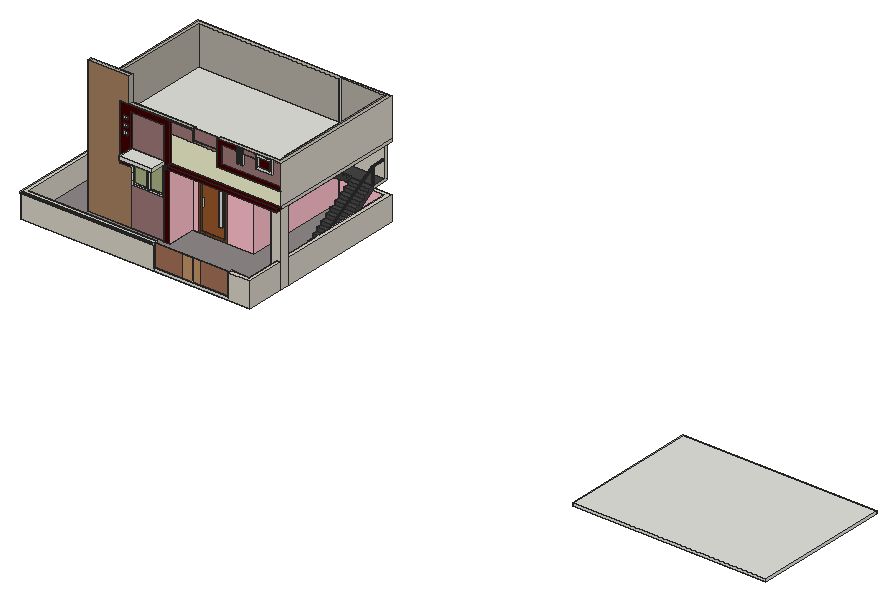
# SketchUp Ruby script. Lengths in inches.
U = 1.inch
M = Sketchup.active_model
def pt(a) = Geom::Point3d.new(a.map { |v| v * U })
def face(e, loops, mat)
  f = e.add_face(loops[0].map { |a| pt(a) })
  loops[1..].each { |l| e.add_face(l.map { |a| pt(a) }).erase! }
  f.material = f.back_material = mat if mat
  f
end
# faces: each face lists its corners as indices into pts; further lists are holes
def faces(e, pts, list, mat = nil) = list.each { |f| face(e, (f[0].is_a?(Array) ? f : [f]).map { |l| l.map { |i| pts[i] } }, mat) }
# xy, xz, yz: faces in a plane at the given z, y or x. An outline is a flat list of corners, or four numbers for a rectangle; further outlines are holes
def ring(l) = l.size == 4 ? [[l[0], l[1]], [l[2], l[1]], [l[2], l[3]], [l[0], l[3]]] : l.each_slice(2).to_a
def flat(e, list, mat, &to3) = list.each { |f| face(e, (f[0].is_a?(Array) ? f : [f]).map { |l| ring(l).map { |u, v| to3.(u, v) } }, mat) }
def xy(e, z, list, mat = nil) = flat(e, list, mat) { |x, y| [x, y, z] }
def xz(e, y, list, mat = nil) = flat(e, list, mat) { |x, z| [x, y, z] }
def yz(e, x, list, mat = nil) = flat(e, list, mat) { |y, z| [x, y, z] }
def lines(e, pts, list) = list.each { |a, b| e.add_line(pt(pts[a]), pt(pts[b])) }
# prism: a flat outline (further loops are holes) pulled along v
def prism(e, loops, v, mat = nil)
  f = face(e, loops, mat); d = Geom::Vector3d.new(v.map { |x| x * U })
  f.pushpull(f.normal.samedirection?(d) ? d.length : -d.length)
end
def box(e, o, s, mat = nil) = prism(e, [[o, [o[0] + s[0], o[1], o[2]], [o[0] + s[0], o[1] + s[1], o[2]], [o[0], o[1] + s[1], o[2]]]], [0, 0, s[2]], mat)
def at(x, y, z, deg = 0) = Geom::Transformation.translation(pt([x, y, z])) * Geom::Transformation.rotation(ORIGIN, Z_AXIS, deg.degrees)
def axes(o, x, y, z) = Geom::Transformation.new([*x, 0, *y, 0, *z, 0, *pt(o).to_a, 1])
def part(name) = M.definitions.add(name)
# library, detail: a bought-in or finely detailed component or shape, given as its bounding box
def library(name, o, s) = part(name).tap { |d| box(d.entities, o, s) }
def detail(e, o, s) = box(e.add_group.entities, o, s)
def put(e, d, t, mat = nil) = e.add_instance(d, t).tap { |i| i.material = mat if mat }
def group(e, t, mat = nil) = e.add_group.tap { |g| g.transformation = t; g.material = mat if mat }.entities
root = M.entities
M.materials.add("[0006_Pink]").color = [255, 192, 203]
M.materials.add("[0022_Maroon]").color = [66, 0, 0]
M.materials.add("[0022_Maroon]1").color = [94, 0, 0]
M.materials.add("[0030_OldLace]").color = [216, 209, 197]
M.materials.add("[0030_OldLace]1").color = [181, 175, 164]
M.materials.add("[0119_RosyBrown]").color = [155, 118, 118]
M.materials.add("[Checker Plate]").color = [242, 245, 207]
M.materials.add("[Cladding Siding Tan]").color = [162, 126, 95]
M.materials.add("[Earth Compacted Fill]").color = [193, 148, 104]
M.materials.add("[Granite Dark Gray]").color = [69, 68, 68]
M.materials.add("[Modern Siding]").color = [160, 111, 84]
M.materials.add("[Stone Marble]").color = [143, 138, 136]
M.materials.add("[Translucent Glass Gray]").color = [115, 128, 45]
M.materials["[Translucent Glass Gray]"].alpha = 0.5
M.materials.add("[Wood Bamboo]").color = [117, 69, 28]
M.materials.add("[Wood Cherry Original]").color = [152, 86, 42]
M.materials.add("[Wood Floor]").color = [155, 105, 61]
xy(root,0,[[0,398.6875,996,1166.6875]])
xy(root,12,[[576,398.6875,900,405.0625],[576,405.0625,900,409.24],[492,561.6875,516,566.6875],[156,566.6875,156,686.6875,174,686.6875,174,584.6875,516,584.6875,516,566.6875],[953.5,566.6875,978,602.6875],
  [174,584.6875,498,686.6875],[498,584.6875,516,686.6875],[156,686.6875,780,1166.6875],[885.375,851.55,978,869.55]])
xy(root,12,[[576,409.24,900,409.24,900,416.6875,978,416.6875,978,566.6875,953.5,566.6875,953.5,602.6875,978,602.6875,978,851.55,885.375,851.55,885.375,869.55,978,869.55,978,1148.6875,780,1148.6875,780,686.6875,516,686.6875,516,561.6875,492,561.6875,492,566.6875,156,566.6875,156,1148.6875,18,1148.6875,18,416.6875,576,416.6875]],"[Stone Marble]")
xy(root,22.43,[[552.2,686.6875,654.59,688.6875]],"[Wood Bamboo]")
xy(root,27.52,[[972.4,855.88,971.62,855.94,970.88,856.2,970.23,856.64,969.73,857.24,969.39,857.94,969.24,858.71,969.3,859.5,969.56,860.23,970.01,860.88,970.6,861.39,971.31,861.73,972.08,861.87,972.86,861.81,973.6,861.55,974.24,861.11,974.75,860.51,975.09,859.81,975.23,859.04,975.17,858.25,974.91,857.52,974.47,856.87,973.875,856.36,973.17,856.02]])
xy(root,27.52,[[[885.375,851.55,978,875.55],[972.4,855.88,971.62,855.94,970.88,856.2,970.23,856.64,969.73,857.24,969.39,857.94,969.24,858.71,969.3,859.5,969.56,860.23,970.01,860.88,970.6,861.39,971.31,861.73,972.08,861.87,972.86,861.81,973.6,861.55,974.24,861.11,974.75,860.51,975.09,859.81,975.23,859.04,975.17,858.25,974.91,857.52,974.47,856.87,973.875,856.36,973.17,856.02]]],"[Granite Dark Gray]")
xy(root,43.03,[[885.375,875.55,978,899.55]],"[Granite Dark Gray]")
xy(root,58.55,[[885.375,899.55,978,923.55]],"[Granite Dark Gray]")
xy(root,63.87,[[630.63,686.6875,644.94,688.6875]])
xy(root,74.07,[[885.375,923.55,978,947.55]],"[Granite Dark Gray]")
xy(root,89.59,[[885.375,947.55,978,971.55]],"[Granite Dark Gray]")
xy(root,102,[[0,394.6875,576,398.6875]])
xy(root,105.1,[[885.375,971.55,978,995.55]],"[Granite Dark Gray]")
xy(root,105.625,[[576,405.0625,900,409.24]])
xy(root,108,[[0,394.6875,576,398.6875]])
xy(root,108,[[0,398.6875,576,398.6875,576,416.6875,18,416.6875,18,1148.6875,156,1148.6875,156,1166.6875,0,1166.6875],[900,398.6875,996,398.6875,996,566.6875,978,566.6875,978,416.6875,900,416.6875],[978,602.6875,996,602.6875,996,1166.6875,780,1166.6875,780,1148.6875,978,1148.6875]],"[0030_OldLace]")
xy(root,115.29,[[559.11,686.6875,561.49,688.6875]])
xy(root,120.62,[[885.375,995.55,978,1019.55]],"[Granite Dark Gray]")
xy(root,136.14,[[885.375,1019.55,978,1043.55]],"[Granite Dark Gray]")
xy(root,151.66,[[885.375,1043.55,978,1067.55]],"[Granite Dark Gray]")
xy(root,152.67,[[559.11,686.6875,561.49,688.6875]])
xy(root,156.83,[[786,1073.55,878.625,1091.55],[780,1091.55,978,1166.6875]])
xy(root,167.17,[[780,1091.55,786,1091.9],[786,1091.55,878.625,1091.9],[969.5625,1094.53,968.8,1094.71,968.11,1095.08,967.54,1095.61,967.125,1096.28,966.9,1097.03,966.87,1097.8125,967.05,1098.57,967.42,1099.26,967.95,1099.84,968.62,1100.25,969.36,1100.48,970.15,1100.5,970.91,1100.33,971.6,1099.96,972.17,1099.42,972.59,1098.76,972.82,1098.01,972.84,1097.23,972.66,1096.46,972.3,1095.77,971.76,1095.2,971.1,1094.79,970.35,1094.56]])
xy(root,167.17,[[885.375,1067.55,978,1091.55],[[878.625,1091.55,978,1091.55,978,1154.6875,780,1154.6875,780,1091.9,878.625,1091.9],[969.5625,1094.53,968.8,1094.71,968.11,1095.08,967.54,1095.61,967.125,1096.28,966.9,1097.03,966.87,1097.8125,967.05,1098.57,967.42,1099.26,967.95,1099.84,968.62,1100.25,969.36,1100.48,970.15,1100.5,970.91,1100.33,971.6,1099.96,972.17,1099.42,972.59,1098.76,972.82,1098.01,972.84,1097.23,972.66,1096.46,972.3,1095.77,971.76,1095.2,971.1,1094.79,970.35,1094.56]]],"[Granite Dark Gray]")
xy(root,172.34,[[786,1091.55,878.625,1091.9]])
xy(root,172.34,[[786,1067.55,878.625,1091.55]],"[Granite Dark Gray]")
xy(root,187.86,[[786,1043.55,878.625,1067.55]],"[Granite Dark Gray]")
xy(root,191.72,[[358.5625,566.6875,412.15,568.6875],[427.85,566.6875,481.4375,568.6875]])
xy(root,203.38,[[786,1019.55,878.625,1043.55]],"[Granite Dark Gray]")
xy(root,209.37,[[630.63,686.6875,644.94,688.6875]])
xy(root,218.9,[[786,995.55,878.625,1019.55]],"[Granite Dark Gray]")
xy(root,234.41,[[786,971.55,878.625,995.55]],"[Granite Dark Gray]")
xy(root,236.26,[[552.2,686.6875,654.59,688.6875]],"[Wood Bamboo]")
xy(root,239.17,[[969.5625,1094.53,970.35,1094.56,971.1,1094.79,971.76,1095.2,972.3,1095.77,972.66,1096.46,972.84,1097.23,972.82,1098.01,972.59,1098.76,972.17,1099.42,971.6,1099.96,970.91,1100.33,970.15,1100.5,969.86,1100.49,969.36,1100.48,968.62,1100.25,967.95,1099.84,967.42,1099.26,967.05,1098.57,966.87,1097.8125,966.9,1097.03,967.125,1096.28,967.54,1095.61,968.11,1095.08,968.8,1094.71]])
xy(root,249.93,[[786,947.55,878.625,971.55]],"[Granite Dark Gray]")
xy(root,252,[[300,561.6875,348,566.6875]],"[0022_Maroon]")
xy(root,265.45,[[786,923.55,878.625,947.55]],"[Granite Dark Gray]")
xy(root,280.97,[[786,899.55,878.625,923.55]],"[Granite Dark Gray]")
xy(root,296.48,[[786,875.55,878.625,899.55]])
xy(root,301.4375,[[358.5625,566.6875,412.15,568.6875],[427.85,566.6875,481.4375,568.6875]])
xy(root,312,[[348,494.6875,492,566.6875],[174,584.6875,498,686.6875],[498,584.6875,516,686.6875],[786,851.55,878.625,875.55]])
xy(root,312,[[516,542.6875,996,566.6875]],"[0022_Maroon]")
xy(root,312,[[516,566.6875,516,686.6875,780,686.6875,780,1154.6875,786,1154.6875,786,851.55,978,851.55,978,1166.6875,996,1166.6875,996,602.6875,953.5,602.6875,953.5,566.6875]],"[Wood Floor]")
xy(root,324,[[348,494.6875,492,566.6875],[174,584.6875,978,584.6875,978,851.55,786,851.55,786,1148.6875,174,1148.6875]])
xy(root,324,[[516,542.6875,996,566.6875]],"[0022_Maroon]")
xy(root,369.54,[[316.43,561.6875,332.18,566.6875]])
xy(root,384,[[720,565.1875,996,566.6875]],"[0022_Maroon]")
xy(root,385.29,[[316.43,561.6875,332.18,566.6875]])
xy(root,399.54,[[316.43,561.6875,332.18,566.6875]])
xy(root,401,[[738,565.1875,996,566.6875]],"[0022_Maroon]")
xy(root,415.29,[[316.43,561.6875,332.18,566.6875]])
xy(root,427.6875,[[804,563.6875,814.375,566.6875],[822,563.6875,832.375,566.6875]])
xy(root,429.54,[[316.43,561.6875,332.18,566.6875]])
xy(root,434.5,[[888,563.6875,960,566.6875]])
xy(root,443.75,[[897.25,563.6875,950.75,566.6875]])
xy(root,445.29,[[316.43,561.6875,332.18,566.6875]])
xy(root,447,[[612,572.9,720,577.76],[612,577.76,720,584.6875]])
xy(root,447,[[612,566.6875,720,572.9]],"[0119_RosyBrown]")
xy(root,468,[[348,561.6875,492,566.6875]])
xy(root,474,[[832.375,565.1875,888,566.6875]])
xy(root,474,[[738,565.1875,804,566.6875]],"[0022_Maroon]")
xy(root,482.75,[[897.25,563.6875,950.75,566.6875]])
xy(root,489,[[516,563.6875,612,566.6875]],"[0119_RosyBrown]")
xy(root,492,[[804,563.6875,814.375,566.6875],[822,563.6875,832.375,566.6875],[888,563.6875,960,566.6875]])
xy(root,492,[[300,561.6875,516,566.6875],[720,565.1875,804,566.6875]],"[0022_Maroon]")
xy(root,492,[[336,566.6875,612,584.6875],[720,566.6875,996,566.6875,996,1166.6875,978,1166.6875,978,584.6875,720,584.6875],[156,584.6875,174,584.6875,174,1148.6875,780,1148.6875,780,1166.6875,156,1166.6875],[780,1148.6875,786,1148.6875,786,1154.6875,978,1154.6875,978,1166.6875,780,1166.6875]],"[0030_OldLace]1")
xy(root,492,[[516,563.6875,612,566.6875],[832.375,565.1875,888,566.6875],[612,572.9,720,577.76]],"[0119_RosyBrown]")
xy(root,600,[[156,566.6875,336,584.6875]],"[0030_OldLace]1")
xz(root,394.6875,[[0,102,576,108]],"[0022_Maroon]1")
xz(root,398.6875,[[576,0,900,12],[0,102,576,108]])
xz(root,398.6875,[[0,0,576,102],[900,0,996,108]],"[0030_OldLace]")
xz(root,405.0625,[[736.23,12,741.15,105.625]])
xz(root,405.0625,[[700.23,12,736.23,105.625],[741.15,12,777.15,105.625]],"[Earth Compacted Fill]")
xz(root,405.0625,[[576,12,700.23,105.625],[777.15,12,900,105.625]],"[Modern Siding]")
xz(root,409.24,[[576,12,900,105.625]],"[Earth Compacted Fill]")
xz(root,416.6875,[[18,12,156,108],[156,12,576,108],[900,12,978,108]])
xz(root,494.6875,[[348,312,492,324]])
xz(root,542.6875,[[516,312,996,324]],"[0022_Maroon]")
xz(root,561.6875,[[[492,12,516,12,516,492,300,492,300,252,348,252,348,468,492,468],[316.43,429.54,332.18,445.29],[316.43,399.54,332.18,415.29],[316.43,369.54,332.18,385.29]]],"[0022_Maroon]")
xz(root,563.6875,[[804,427.6875,814.375,492],[822,427.6875,832.375,492],[[888,434.5,960,492],[897.25,443.75,950.75,482.75]]])
xz(root,563.6875,[[516,489,612,492]],"[0119_RosyBrown]")
xz(root,565.1875,[[720,384,996,384,996,401,738,401,738,474,804,474,804,492,720,492]],"[0022_Maroon]")
xz(root,565.1875,[[832.375,474,888,492]],"[0119_RosyBrown]")
xz(root,566.6875,[[978,12,996,108],[348,181.16,416,181.16,416,187.87,354.71,187.87,354.71,305.29,485.29,305.29,485.29,187.87,424,187.87,424,181.16,492,181.16,492,312,348,312],[416,181.16,424,187.87],[[354.71,187.87,416,305.29],[358.5625,191.72,412.15,301.4375]],[416,187.87,424,305.29],
  [[424,187.87,485.29,305.29],[427.85,191.72,481.4375,301.4375]],[348,312,492,324],[516,312,996,324],[316.43,369.54,332.18,385.29],[720,384,720,492,804,492,804,474,738,474,738,401,996,401,996,384],
  [316.43,399.54,332.18,415.29],[804,427.6875,814.375,492],[822,427.6875,832.375,492],[316.43,429.54,332.18,445.29],[[888,434.5,960,492],[897.25,443.75,950.75,482.75]],
  [832.375,474,888,492],[516,489,612,492]])
xz(root,566.6875,[[897.25,443.75,950.75,482.75]],"[0022_Maroon]")
xz(root,566.6875,[[953.5,12,978,12,978,108,996,108,996,312,953.5,312]],"[0030_OldLace]")
xz(root,566.6875,[[348,12,492,181.16],[348,324,492,468],[738,401,996,401,996,492,960,492,960,434.5,888,434.5,888,474,832.375,474,832.375,427.6875,822,427.6875,822,474,814.375,474,814.375,427.6875,804,427.6875,804,474,738,474],[516,438,720,438,720,447,612,447,612,489,516,489],[814.375,474,822,492]],"[0119_RosyBrown]")
xz(root,566.6875,[[516,324,996,324,996,384,720,384,720,438,516,438]],"[Checker Plate]")
xz(root,566.6875,[[156,12,348,12,348,252,300,252,300,492,336,492,336,600,156,600]],"[Cladding Siding Tan]")
xz(root,568.6875,[[358.5625,191.72,412.15,301.4375],[427.85,191.72,481.4375,301.4375]],"[Translucent Glass Gray]")
xz(root,572.9,[[612,447,720,492]],"[0119_RosyBrown]")
xz(root,577.76,[[612,447,720,492]])
xz(root,584.6875,[[174,12,498,312]])
xz(root,584.6875,[[174,324,174,600,336,600,336,492,612,492,612,447,720,447,720,492,978,492,978,324],[156,492,174,600]],"[0030_OldLace]1")
xz(root,602.6875,[[953.5,12,953.5,312,996,312,996,108,978,108,978,12],[978,12,996,108]])
xz(root,686.6875,[[174,12,498,312],[498,12,516,312],[630.63,63.87,644.94,209.37],[559.11,115.29,561.49,152.67]])
xz(root,686.6875,[[516,12,541.77,12,541.77,246.6875,665.02,246.6875,665.02,12,780,12,780,312,516,312]],"[0006_Pink]")
xz(root,686.6875,[[[541.77,12,665.02,246.6875],[552.2,22.43,654.59,236.26]]],"[Wood Bamboo]")
xz(root,688.6875,[[[552.2,22.43,654.59,236.26],[630.63,63.87,644.94,209.37],[559.11,115.29,561.49,152.67]]],"[Wood Cherry Original]")
xz(root,851.55,[[786,312,978,324]])
xz(root,851.55,[[786,301.66,878.625,312]],"[0006_Pink]")
xz(root,851.55,[[885.375,12,978,27.52]],"[Granite Dark Gray]")
xz(root,875.55,[[885.375,27.52,978,43.03],[786,296.48,878.625,312]],"[Granite Dark Gray]")
xz(root,899.55,[[885.375,43.03,978,58.55],[786,280.97,878.625,296.48]],"[Granite Dark Gray]")
xz(root,923.55,[[885.375,58.55,978,74.07],[786,265.45,878.625,280.97]],"[Granite Dark Gray]")
xz(root,947.55,[[885.375,74.07,978,89.59],[786,249.93,878.625,265.45]],"[Granite Dark Gray]")
xz(root,971.55,[[885.375,89.59,978,105.1],[786,234.41,878.625,249.93]],"[Granite Dark Gray]")
xz(root,995.55,[[885.375,105.1,978,120.62],[786,218.9,878.625,234.41]],"[Granite Dark Gray]")
xz(root,1019.55,[[885.375,120.62,978,136.14],[786,203.38,878.625,218.9]],"[Granite Dark Gray]")
xz(root,1043.55,[[885.375,136.14,978,151.66],[786,187.86,878.625,203.38]],"[Granite Dark Gray]")
xz(root,1067.55,[[885.375,151.66,978,167.17],[786,172.34,878.625,187.86]],"[Granite Dark Gray]")
xz(root,1091.55,[[780,156.83,786,167.17],[786,156.83,878.625,167.17],[878.625,156.83,885.375,167.17],[885.375,156.83,978,167.17],[786,167.17,878.625,172.34]])
xz(root,1091.9,[[786,167.17,878.625,172.34]])
xz(root,1148.6875,[[780,324,786,492]])
xz(root,1148.6875,[[780,12,978,108]],"[0006_Pink]")
xz(root,1148.6875,[[18,12,156,108]],"[0030_OldLace]")
xz(root,1148.6875,[[174,324,780,492]],"[0030_OldLace]1")
xz(root,1154.6875,[[969.86,236.17,970.18,236.21,969.79,236.18],[969.4,236.23,969.01,236.3,969.08,236.27],[970.5625,236.27,970.63,236.27,970.93,236.4],[968.65,236.45,968.3,236.62,968.36,236.57],[971.29,236.55,971.36,236.57,971.61,236.77],
  [967.99,236.85,967.69,237.11,967.73,237.05],[971.92,237.01,971.98,237.05,972.17,237.31],[967.45,237.42,967.23,237.74,967.26,237.67],[972.41,237.62,972.45,237.67,972.58,237.97],[967.08,238.1,966.95,238.47,966.96,238.4],
  [972.73,238.33,972.75,238.4,972.8,238.72],[966.9,238.85,966.86,239.24,966.86,239.17],[972.85,239.1,972.86,239.17,972.8125,239.49],[966.92,239.63,966.98,240.01,966.96,239.95],[972.76,239.88,972.75,239.95,972.63,240.25],
  [967.13,240.375,967.3,240.73,967.26,240.67],[972.48,240.61,972.45,240.67,972.26,240.93],[967.54,241.04,967.79,241.34,967.73,241.29],[972.02,241.24,971.98,241.29,971.72,241.49],[968.1,241.57,968.42,241.8,968.36,241.77],
  [971.41,241.73,971.36,241.77,971.06,241.89],[968.78,241.95,969.15,242.08,969.08,242.07],[970.7,242.04,970.63,242.07,970.3125,242.11],[969.54,242.13,969.92,242.16,969.86,242.17]])
xz(root,1154.6875,[[[780,167.17,978,167.17,978,324,786,324,786,312,780,312],[969.86,236.17,969.79,236.18,969.72,236.18,969.4,236.23,969.08,236.27,969.01,236.3,968.95,236.3125,968.65,236.45,968.36,236.57,968.3,236.62,968.24,236.65,967.99,236.85,967.73,237.05,967.69,237.11,967.64,237.15,967.45,237.42,967.26,237.67,967.23,237.74,967.19,237.79,967.08,238.1,966.96,238.4,966.95,238.47,966.93,238.53,966.9,238.85,966.86,239.17,966.86,239.3125,966.92,239.63,966.96,239.95,966.98,240.01,967,240.08,967.26,240.67,967.3,240.73,967.33,240.79,967.54,241.04,967.73,241.29,967.79,241.34,967.83,241.39,968.1,241.57,968.36,241.77,968.42,241.8,968.48,241.84,968.78,241.95,969.08,242.07,969.15,242.08,969.21,242.1,969.54,242.13,969.86,242.17,969.92,242.16,969.99,242.17,970.3125,242.11,970.63,242.07,970.7,242.04,970.77,242.03,971.06,241.89,971.36,241.77,971.41,241.73,971.47,241.7,971.72,241.49,971.98,241.29,972.02,241.24,972.07,241.19,972.45,240.67,972.48,240.61,972.52,240.55,972.63,240.25,972.75,239.95,972.76,239.88,972.79,239.8125,972.8125,239.49,972.86,239.17,972.85,239.1,972.85,239.03,972.8,238.72,972.75,238.4,972.71,238.26,972.58,237.97,972.45,237.67,972.41,237.62,972.38,237.55,972.17,237.31,971.98,237.05,971.92,237.01,971.875,236.96,971.61,236.77,971.36,236.57,971.29,236.55,971.23,236.51,970.93,236.4,970.63,236.27,970.5625,236.27,970.5,236.24,970.18,236.21]]],"[0030_OldLace]")
xz(root,1154.6875,[[786,324,978,492]],"[0030_OldLace]1")
xz(root,1166.6875,[[0,0,156,12],[156,0,996,12],[0,12,156,108],[156,12,780,492],[780,12,996,108],
  [780,156.83,978,492],[978,312,996,492]],"[0030_OldLace]")
yz(root,0,[[394.6875,102,398.6875,108]])
yz(root,0,[[398.6875,0,1166.6875,108]],"[0030_OldLace]")
yz(root,18,[[416.6875,12,1148.6875,108]],"[0030_OldLace]")
yz(root,156,[[1148.6875,12,1166.6875,108],[566.6875,492,584.6875,600]])
yz(root,156,[[566.6875,12,566.6875,492,1166.6875,492,1166.6875,108,1148.6875,108,1148.6875,12]],"[0030_OldLace]")
yz(root,174,[[584.6875,12,686.6875,312]])
yz(root,174,[[584.6875,324,1148.6875,492]],"[0030_OldLace]1")
yz(root,300,[[561.6875,252,566.6875,492]],"[0022_Maroon]")
yz(root,316.43,[[561.6875,369.54,566.6875,385.29],[561.6875,399.54,566.6875,415.29],[561.6875,429.54,566.6875,445.29]])
yz(root,332.18,[[561.6875,369.54,566.6875,385.29],[561.6875,399.54,566.6875,415.29],[561.6875,429.54,566.6875,445.29]])
yz(root,336,[[566.6875,492,584.6875,600]],"[0030_OldLace]1")
yz(root,348,[[561.6875,252,566.6875,312],[494.6875,312,561.6875,324],[561.6875,312,566.6875,324]])
yz(root,348,[[561.6875,324,566.6875,468]],"[0022_Maroon]")
yz(root,358.5625,[[566.6875,191.72,568.6875,252],[566.6875,252,568.6875,301.4375]])
yz(root,412.15,[[566.6875,191.72,568.6875,301.4375]])
yz(root,427.85,[[566.6875,191.72,568.6875,301.4375]])
yz(root,481.4375,[[566.6875,191.72,568.6875,301.4375]])
yz(root,492,[[494.6875,312,561.6875,324],[561.6875,312,566.6875,324]])
yz(root,492,[[561.6875,12,566.6875,312],[561.6875,324,566.6875,468]],"[0022_Maroon]")
yz(root,498,[[584.6875,12,686.6875,312]])
yz(root,516,[[561.6875,312,566.6875,324],[563.6875,489,566.6875,492]])
yz(root,516,[[561.6875,12,686.6875,312]],"[0006_Pink]")
yz(root,516,[[542.6875,312,561.6875,324],[561.6875,324,566.6875,324,566.6875,489,563.6875,489,563.6875,492,561.6875,492]],"[0022_Maroon]")
yz(root,552.2,[[686.6875,22.43,688.6875,236.26]],"[Wood Bamboo]")
yz(root,559.11,[[686.6875,115.29,688.6875,152.67]])
yz(root,561.49,[[686.6875,115.29,688.6875,152.67]])
yz(root,576,[[398.6875,12,405.0625,12,405.0625,105.625,409.24,105.625,409.24,12,416.6875,12,416.6875,108,398.6875,108],[405.0625,12,409.24,105.625],[394.6875,102,398.6875,108]])
yz(root,612,[[572.9,447,577.76,492],[577.76,447,584.6875,492]])
yz(root,612,[[566.6875,447,572.9,492],[563.6875,489,566.6875,492]],"[0119_RosyBrown]")
yz(root,630.63,[[686.6875,63.87,688.6875,209.37]])
yz(root,644.94,[[686.6875,63.87,688.6875,209.37]])
yz(root,654.59,[[686.6875,22.43,688.6875,236.26]],"[Wood Bamboo]")
yz(root,720,[[566.6875,447,572.9,492],[572.9,447,577.76,492],[577.76,447,584.6875,492]])
yz(root,720,[[565.1875,384,565.1875,444,566.6875,438,566.6875,384],[566.6875,438,565.1875,444,565.1875,492,566.6875,492]],"[0022_Maroon]")
yz(root,738,[[565.1875,401,566.6875,468],[565.1875,468,566.6875,474]],"[0022_Maroon]")
yz(root,780,[[1148.6875,12,1166.6875,108],[1148.6875,324,1166.6875,492]])
yz(root,780,[[686.6875,12,1148.6875,12,1148.6875,108,1166.6875,108,1166.6875,156.83,1091.55,156.83,1091.55,167.17,1154.6875,167.17,1154.6875,312,686.6875,312]],"[0006_Pink]")
yz(root,786,[[1073.55,156.83,851.55,301.66,851.55,312,875.55,312,875.55,296.48,899.55,296.48,899.55,280.97,923.55,280.97,923.55,265.45,947.55,265.45,947.55,249.93,971.55,249.93,971.55,234.41,995.55,234.41,995.55,218.9,1019.55,218.9,1019.55,203.38,1043.55,203.38,1043.55,187.86,1067.55,187.86,1067.55,172.34,1091.55,172.34,1091.55,156.83],[1091.55,167.17,1091.9,172.34],[851.55,312,1154.6875,324],[1148.6875,324,1154.6875,492]])
yz(root,804,[[563.6875,427.6875,563.6875,492,565.1875,492,565.1875,474,566.6875,474,566.6875,427.6875],[565.1875,474,566.6875,492]])
yz(root,814.375,[[563.6875,427.6875,566.6875,492]])
yz(root,822,[[563.6875,427.6875,566.6875,492]])
yz(root,832.375,[[563.6875,427.6875,566.6875,427.6875,566.6875,474,565.1875,474,565.1875,492,563.6875,492],[565.1875,474,566.6875,492]])
yz(root,878.625,[[1091.55,167.17,1091.9,172.34]])
yz(root,878.625,[[1073.55,156.83,1091.55,156.83,1091.55,172.34,1067.55,172.34,1067.55,187.86,1043.55,187.86,1043.55,203.38,1019.55,203.38,1019.55,218.9,995.55,218.9,995.55,234.41,971.55,234.41,971.55,249.93,947.55,249.93,947.55,265.45,923.55,265.45,923.55,280.97,899.55,280.97,899.55,296.48,875.55,296.48,875.55,312,851.55,312,851.55,301.66]],"[Granite Dark Gray]")
yz(root,885.375,[[851.55,12,851.55,27.52,875.55,27.52,875.55,43.03,899.55,43.03,899.55,58.55,923.55,58.55,923.55,74.07,947.55,74.07,947.55,89.59,971.55,89.59,971.55,105.1,995.55,105.1,995.55,120.62,1019.55,120.62,1019.55,136.14,1043.55,136.14,1043.55,151.66,1067.55,151.66,1067.55,167.17,1091.55,167.17,1091.55,156.83,869.55,12]],"[Granite Dark Gray]")
yz(root,888,[[563.6875,434.5,563.6875,492,565.1875,492,565.1875,474,566.6875,474,566.6875,434.5],[565.1875,474,566.6875,492]])
yz(root,897.25,[[563.6875,443.75,566.6875,482.75]])
yz(root,900,[[398.6875,12,398.6875,108,416.6875,108,416.6875,12,409.24,12,409.24,105.625,405.0625,105.625,405.0625,12],[405.0625,12,409.24,105.625]])
yz(root,950.75,[[563.6875,443.75,566.6875,482.75]])
yz(root,953.5,[[566.6875,12,602.6875,312]])
yz(root,960,[[563.6875,434.5,566.6875,492]])
yz(root,978,[[416.6875,12,566.6875,108],[602.6875,12,851.55,108],[851.55,12,869.55,27.52],[869.55,12,1016.71,108,1148.6875,108,1148.6875,12],[869.55,12,1016.71,108,995.55,108,995.55,105.1,971.55,105.1,971.55,89.59,947.55,89.59,947.55,74.07,923.55,74.07,923.55,58.55,899.55,58.55,899.55,43.03,875.55,43.03,875.55,27.52,869.55,27.52],
  [851.55,27.52,869.55,108],[869.55,27.52,869.55,108,995.55,108,995.55,105.1,971.55,105.1,971.55,89.59,947.55,89.59,947.55,74.07,923.55,74.07,923.55,58.55,899.55,58.55,899.55,43.03,875.55,43.03,875.55,27.52],[1154.6875,312,1166.6875,324],[1154.6875,324,1163.55,492],[1163.55,324,1166.6875,492]])
yz(root,978,[[1091.55,156.83,1166.6875,156.83,1166.6875,312,1154.6875,312,1154.6875,167.17,1091.55,167.17]],"[0030_OldLace]")
yz(root,978,[[851.55,312,1154.6875,324],[584.6875,324,1148.6875,492],[1148.6875,324,1154.6875,492]],"[0030_OldLace]1")
yz(root,978,[[995.55,108,1016.71,108,1091.55,156.83,1091.55,167.17,1067.55,167.17,1067.55,151.66,1043.55,151.66,1043.55,136.14,1019.55,136.14,1019.55,120.62,995.55,120.62]],"[Granite Dark Gray]")
yz(root,996,[[565.1875,384,566.6875,401]])
yz(root,996,[[542.6875,312,566.6875,324]],"[0022_Maroon]")
yz(root,996,[[398.6875,0,566.6875,108],[566.6875,0,602.6875,312],[602.6875,0,1166.6875,108],[566.6875,312,1166.6875,324],[566.6875,324,1166.6875,492]],"[0030_OldLace]")
p = [[978,1016.71,108],[978,869.55,12],[885.375,869.55,12],[885.375,1091.55,156.83],[978,1091.55,156.83],[970.88,856.2,27.52],
  [971.62,855.94,27.52],[971.62,855.94,101.2],[970.88,856.2,101.04],[972.4,855.88,27.52],[972.4,855.88,101.24],[973.17,856.02,27.52],
  [973.17,856.02,101.16],[973.875,856.36,27.52],[973.875,856.36,100.97],[970.23,856.64,27.52],[970.23,856.64,100.79],[974.47,856.87,27.52],
  [974.47,856.87,100.68],[969.73,857.24,27.52],[969.73,857.24,100.44],[974.91,857.52,27.52],[974.91,857.52,100.3125],[969.39,857.94,27.52],
  [969.39,857.94,100.03],[975.17,858.25,27.52],[975.17,858.25,99.89],[969.24,858.71,27.52],[969.24,858.71,99.59],[975.23,859.04,27.52],
  [975.23,859.04,99.44],[969.3,859.5,27.52],[969.3,859.5,99.14],[975.09,859.81,27.52],[975.09,859.81,99],[969.56,860.23,27.52],
  [969.56,860.23,98.72],[974.75,860.51,27.52],[974.75,860.51,98.59],[970.01,860.88,27.52],[970.01,860.88,98.35],[974.24,861.11,27.52],
  [974.24,861.11,98.25],[970.6,861.39,27.52],[970.6,861.39,98.07],[973.6,861.55,27.52],[973.6,861.55,97.99],[971.31,861.73,27.52],
  [971.31,861.73,97.875],[972.86,861.81,27.52],[972.86,861.81,97.84],[972.08,861.87,27.52],[972.08,861.87,97.8],[970.5,1098.32,236.24],
  [971.23,1098.25,236.51],[968.95,1098.29,236.3125],[969.72,1098.33,236.18],[968.24,1098.2,236.65],[971.875,1098.13,236.96],[967.64,1098.06,237.15],
  [972.38,1097.97,237.55],[967.19,1097.88,237.79],[972.71,1097.78,238.26],[966.93,1097.68,238.53],[972.85,1097.57,239.03],[966.86,1097.47,239.3125],
  [972.79,1097.36,239.8125],[967,1097.26,240.08],[972.52,1097.16,240.55],[967.33,1097.07,240.79],[972.07,1096.98,241.19],[967.83,1096.91,241.39],
  [971.47,1096.84,241.7],[968.48,1096.79,241.84],[969.21,1096.72,242.1],[970.77,1096.75,242.03],[969.99,1096.71,242.17],[786,851.55,301.66],
  [786,1073.55,156.83],[878.625,1073.55,156.83],[878.625,851.55,301.66],[968.8,1094.71,167.17],[969.5625,1094.53,167.17],[969.5625,1094.53,239.17],
  [968.8,1094.71,239.17],[970.35,1094.56,167.17],[970.35,1094.56,239.17],[971.1,1094.79,167.17],[971.1,1094.79,239.17],[968.11,1095.08,167.17],
  [968.11,1095.08,239.17],[971.76,1095.2,167.17],[971.76,1095.2,239.17],[967.54,1095.61,167.17],[967.54,1095.61,239.17],[972.3,1095.77,167.17],
  [972.3,1095.77,239.17],[967.125,1096.28,167.17],[967.125,1096.28,239.17],[972.66,1096.46,167.17],[972.66,1096.46,239.17],[966.9,1097.03,167.17],
  [966.9,1097.03,239.17],[972.84,1097.23,167.17],[972.84,1097.23,239.17],[966.87,1097.8125,167.17],[966.87,1097.8125,239.17],[972.82,1098.01,167.17],
  [972.82,1098.01,239.17],[967.05,1098.57,167.17],[967.05,1098.57,239.17],[972.59,1098.76,167.17],[972.59,1098.76,239.17],[967.42,1099.26,167.17],
  [967.42,1099.26,239.17],[972.17,1099.42,167.17],[972.17,1099.42,239.17],[967.95,1099.84,167.17],[967.95,1099.84,239.17],[971.6,1099.96,167.17],
  [971.6,1099.96,239.17],[968.62,1100.25,167.17],[968.62,1100.25,239.17],[970.91,1100.33,167.17],[970.91,1100.33,239.17],[969.36,1100.48,167.17],
  [969.36,1100.48,239.17],[970.15,1100.5,167.17],[970.15,1100.5,239.17],[969.86,1100.49,239.17],[970.5,1154.6875,236.24],[970.5625,1154.6875,236.27],
  [970.93,1154.6875,236.4],[971.23,1154.6875,236.51],[968.95,1154.6875,236.3125],[969.01,1154.6875,236.3],[969.4,1154.6875,236.23],[969.72,1154.6875,236.18],
  [969.79,1154.6875,236.18],[970.18,1154.6875,236.21],[968.24,1154.6875,236.65],[968.3,1154.6875,236.62],[968.65,1154.6875,236.45],[971.29,1154.6875,236.55],
  [971.61,1154.6875,236.77],[971.875,1154.6875,236.96],[967.64,1154.6875,237.15],[967.69,1154.6875,237.11],[967.99,1154.6875,236.85],[971.92,1154.6875,237.01],
  [972.17,1154.6875,237.31],[972.38,1154.6875,237.55],[967.19,1154.6875,237.79],[967.23,1154.6875,237.74],[967.45,1154.6875,237.42],[972.41,1154.6875,237.62],
  [972.58,1154.6875,237.97],[972.71,1154.6875,238.26],[966.93,1154.6875,238.53],[966.95,1154.6875,238.47],[967.08,1154.6875,238.1],[972.73,1154.6875,238.33],
  [972.8,1154.6875,238.72],[972.85,1154.6875,239.03],[966.86,1154.6875,239.3125],[966.86,1154.6875,239.24],[966.9,1154.6875,238.85],[972.85,1154.6875,239.1],
  [972.8125,1154.6875,239.49],[972.79,1154.6875,239.8125],[967,1154.6875,240.08],[966.98,1154.6875,240.01],[966.92,1154.6875,239.63],[972.76,1154.6875,239.88],
  [972.63,1154.6875,240.25],[972.52,1154.6875,240.55],[967.33,1154.6875,240.79],[967.3,1154.6875,240.73],[967.13,1154.6875,240.375],[972.48,1154.6875,240.61],
  [972.26,1154.6875,240.93],[972.07,1154.6875,241.19],[967.83,1154.6875,241.39],[967.79,1154.6875,241.34],[967.54,1154.6875,241.04],[972.02,1154.6875,241.24],
  [971.72,1154.6875,241.49],[971.47,1154.6875,241.7],[968.48,1154.6875,241.84],[968.42,1154.6875,241.8],[968.1,1154.6875,241.57],[971.41,1154.6875,241.73],
  [971.06,1154.6875,241.89],[970.77,1154.6875,242.03],[969.21,1154.6875,242.1],[969.15,1154.6875,242.08],[968.78,1154.6875,241.95],[970.7,1154.6875,242.04],
  [970.3125,1154.6875,242.11],[969.99,1154.6875,242.17],[969.92,1154.6875,242.16],[969.54,1154.6875,242.13],[780,1166.6875,312],[780,1154.6875,312],
  [174,686.6875,312],[156,686.6875,312],[174,584.6875,324],[156,584.6875,324],[516,566.6875,324],[516,584.6875,324],
  [780,1163.55,167.17],[978,1163.55,167.17],[780,1163.55,156.83],[780,1154.6875,167.17],[972.24,858.875,27.52],[972.24,858.875,99.52],
  [969.86,1097.52,167.17],[969.86,1097.52,239.17],[969.86,1154.6875,239.17]]
faces(root,p,[[0,1,2,3,4],[5,6,7,8],[6,9,10,7],[9,11,12,10],[11,13,14,12],[15,5,8,16],[13,17,18,14],[19,15,16,20],
  [17,21,22,18],[23,19,20,24],[21,25,26,22],[27,23,24,28],[25,29,30,26],[31,27,28,32],[29,33,34,30],[35,31,32,36],
  [33,37,38,34],[39,35,36,40],[37,41,42,38],[43,39,40,44],[41,45,46,42],[47,43,44,48],[45,49,50,46],[51,47,48,52],
  [49,51,52,50],[46,50,53,54],[52,48,55,56],[50,52,56,53],[48,44,57,55],[42,46,54,58],[44,40,59,57],[38,42,58,60],
  [40,36,61,59],[34,38,60,62],[36,32,63,61],[30,34,62,64],[32,28,65,63],[26,30,64,66],[28,24,67,65],[22,26,66,68],
  [24,20,69,67],[18,22,68,70],[20,16,71,69],[14,18,70,72],[16,8,73,71],[8,7,74,73],[12,14,72,75],[7,10,76,74],
  [10,12,75,76],[81,82,83,84],[82,85,86,83],[85,87,88,86],[89,81,84,90],[87,91,92,88],[93,89,90,94],[91,95,96,92],
  [97,93,94,98],[95,99,100,96],[101,97,98,102],[99,103,104,100],[105,101,102,106],[103,107,108,104],[109,105,106,110],[107,111,112,108],
  [113,109,110,114],[111,115,116,112],[117,113,114,118],[115,119,120,116],[121,117,118,122],[119,123,124,120],[125,121,122,126],[123,127,128,124],
  [127,125,126,129,128],[54,53,130,131,132,133],[56,55,134,135,136,137],[53,56,137,138,139,130],[55,57,140,141,142,134],[58,54,133,143,144,145],[57,59,146,147,148,140],[60,58,145,149,150,151],
  [59,61,152,153,154,146],[62,60,151,155,156,157],[61,63,158,159,160,152],[64,62,157,161,162,163],[63,65,164,165,166,158],[66,64,163,167,168,169],[65,67,170,171,172,164],[68,66,169,173,174,175],
  [67,69,176,177,178,170],[70,68,175,179,180,181],[69,71,182,183,184,176],[72,70,181,185,186,187],[71,73,188,189,190,182],[75,72,187,191,192,193],[73,74,194,195,196,188],[76,75,193,197,198,199],
  [74,76,199,200,201,194]])
faces(root,p,[[77,78,79,80]],"[0006_Pink]")
lines(root,p,[[202,203],[204,205],[206,207],[208,209],[210,211],[210,212],[213,210],[214,215],[216,217],[217,129],[217,215],[129,218]])
g1 = group(root,at(2717.375,0,12))
box(g1,[0,0,0],[840,600,12])
